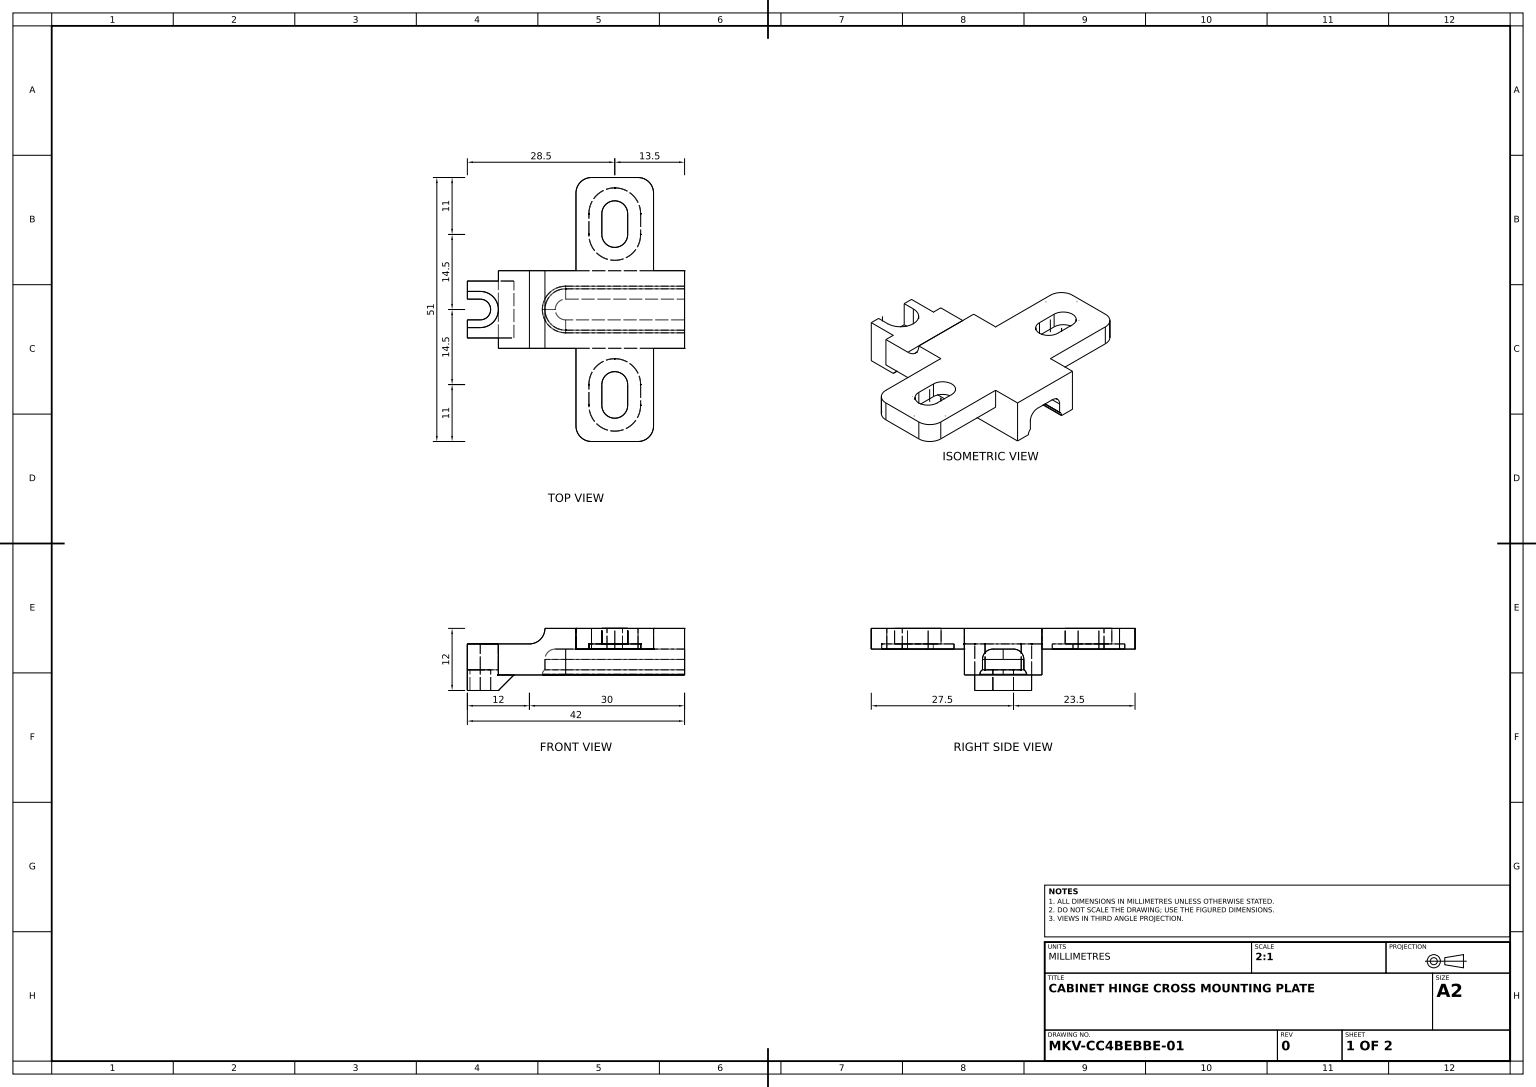
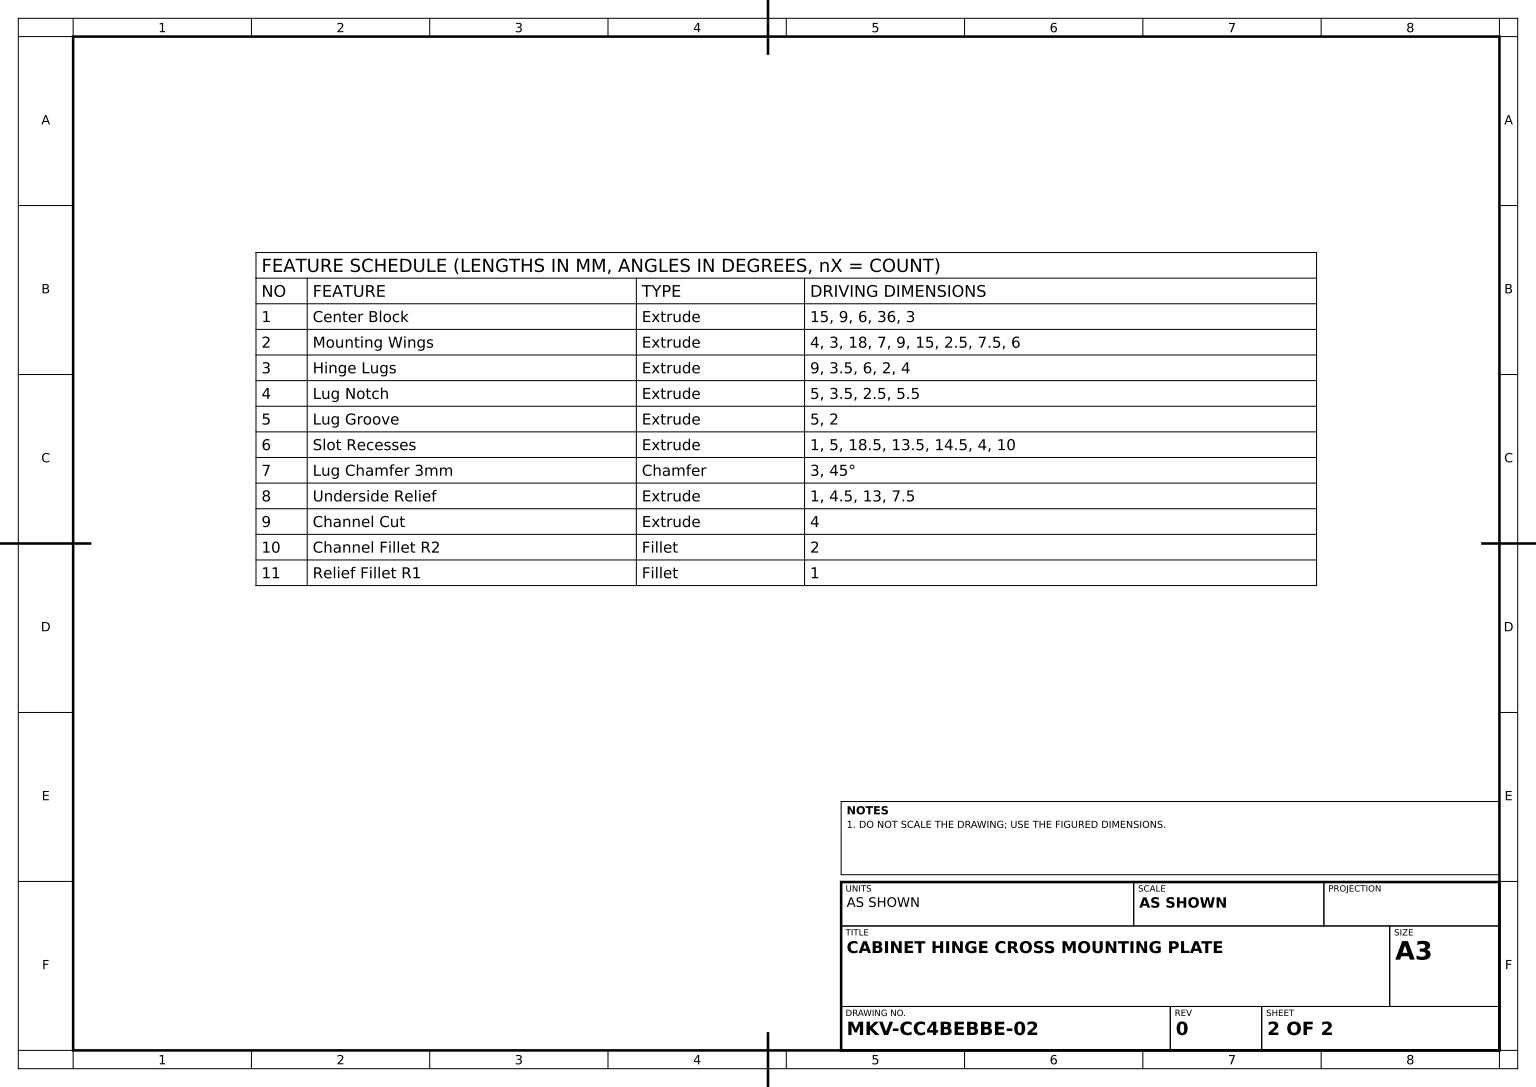
solid
v1 (-8.5,-4,18.5)
v2 (-18.5,-4,18.5)
e1 v1 v2 CIRCLE(AX(P(-13.5,-4,18.5),D(0,-1,0),D(0,0,1)),5)
v3 (-18.5,-3,18.5)
e2 v3 v2 LINE
v4 (-8.5,-3,18.5)
e3 v4 v3 CIRCLE(AX(P(-13.5,-3,18.5),D(0,-1,0),D(0,0,1)),5)
e4 v4 v1 LINE
face CYL(AX(P(-13.5,-3,18.5),D(0,-1,0),D(0,0,-1)),5) rev [e1 -e2 -e3 e4]
v5 (-9,-4,-25.5)
v6 (-18,-4,-25.5)
e5 v5 v6 LINE
v7 (-18,0,-25.5)
e6 v6 v7 LINE
v8 (-9,0,-25.5)
e7 v8 v7 LINE
e8 v5 v8 LINE
face PLANE(AX(P(-18,-4,-25.5),D(0,0,-1),D(-1,0,0))) [e5 e6 -e7 -e8]
v9 (-39.5,-8,2)
v10 (-39.5,-8,-2)
e9 v9 v10 CIRCLE(AX(P(-39.5,-8,0),D(0,1,0),D(0,0,1)),2)
v11 (-42,-8,2)
e10 v11 v9 LINE
v12 (-42,-8,3.5)
e11 v11 v12 LINE
v13 (-39.5,-8,3.5)
e12 v12 v13 LINE
v14 (-39.5,-8,-3.5)
e13 v13 v14 CIRCLE(AX(P(-39.5,-8,0),D(0,1,0),D(0,0,1)),3.5)
v15 (-42,-8,-3.5)
e14 v14 v15 LINE
v16 (-42,-8,-2)
e15 v15 v16 LINE
e16 v10 v16 LINE
face PLANE(AX(P(-39.5,-8,0),D(0,1,0),D(0,0,1))) [-e9 -e10 e11 e12 e13 e14 e15 -e16]
v17 (0,-8,-4)
v18 (0,-8.866025,-4.5)
e17 v17 v18 CIRCLE(AX(P(0,-8.866025,-3.5),D(-1,0,0),D(0,-1,0)),1)
v19 (-23,-8,-4)
e18 v19 v17 LINE
v20 (-23,-8.866025,-4.5)
e19 v20 v19 CIRCLE(AX(P(-23,-8.866025,-3.5),D(1,0,0),D(0,0,-1)),1)
e20 v18 v20 LINE
face CYL(AX(P(-23,-8.866025,-3.5),D(1,0,0),D(0,1,0)),1) rev [-e17 -e18 -e19 -e20]
v21 (-8.5,-4,14.5)
e21 v21 v1 LINE
v22 (-8.5,-3,14.5)
e22 v22 v4 LINE
e23 v22 v21 LINE
face PLANE(AX(P(-8.5,-3,14.5),D(1,0,0),D(0,0,-1))) rev [e21 -e4 -e22 e23]
v23 (-6,-4,-7.5)
v24 (-6,0,-7.5)
e24 v23 v24 LINE
v25 (0,0,-7.5)
e25 v25 v24 LINE
v26 (0,-9,-7.5)
e26 v26 v25 LINE
v27 (-36,-9,-7.5)
e27 v27 v26 LINE
v28 (-36,-3,-7.5)
e28 v28 v27 LINE
v29 (-30,-3,-7.5)
e29 v29 v28 LINE
v30 (-27,0,-7.5)
e30 v30 v29 CIRCLE(AX(P(-30,0,-7.5),D(0,0,-1),D(1,0,0)),3)
v31 (-21,0,-7.5)
e31 v31 v30 LINE
v32 (-21,-4,-7.5)
e32 v32 v31 LINE
e33 v32 v23 LINE
face PLANE(AX(P(-30,0,-7.5),D(0,0,1),D(1,0,0))) rev [e24 -e25 -e26 -e27 -e28 -e29 -e30 -e31 -e32 e33]
v33 (-11,-3,14.5)
v34 (-11,0,14.5)
e34 v33 v34 LINE
v35 (-11,-3,18.5)
e35 v33 v35 LINE
v36 (-11,0,18.5)
e36 v35 v36 LINE
e37 v36 v34 LINE
face PLANE(AX(P(-11,-4,18.5),D(1,0,0),D(0,0,-1))) rev [-e34 e35 e36 e37]
v37 (-8.5,-3,-14.5)
v38 (-18.5,-3,-14.5)
e38 v37 v38 CIRCLE(AX(P(-13.5,-3,-14.5),D(0,-1,0),D(0,0,-1)),5)
v39 (-8.5,-4,-14.5)
e39 v37 v39 LINE
v40 (-18.5,-4,-14.5)
e40 v39 v40 CIRCLE(AX(P(-13.5,-4,-14.5),D(0,-1,0),D(0,0,-1)),5)
e41 v38 v40 LINE
face CYL(AX(P(-13.5,-3,-14.5),D(0,-1,0),D(0,0,-1)),5) rev [-e38 e39 e40 -e41]
v41 (-23,-9,-4.5)
e42 v20 v41 LINE
v42 (0,-9,-4.5)
e43 v41 v42 LINE
e44 v18 v42 LINE
face PLANE(AX(P(0,-8,-4.5),D(0,0,-1),D(-1,0,0))) rev [e42 e43 -e44 e20]
v43 (-16,-3,-14.5)
v44 (-16,0,-14.5)
e45 v43 v44 LINE
v45 (-13.5,0,-12)
e46 v44 v45 CIRCLE(AX(P(-13.5,0,-14.5),D(0,1,0),D(0,0,1)),2.5)
v46 (-13.5,-3,-12)
e47 v46 v45 LINE
e48 v43 v46 CIRCLE(AX(P(-13.5,-3,-14.5),D(0,1,0),D(0,0,-1)),2.5)
face CYL(AX(P(-13.5,-4,-14.5),D(0,1,0),D(0,0,1)),2.5) rev [e45 e46 -e47 -e48]
v47 (0,-6,-4)
e49 v47 v17 LINE
e50 v42 v26 LINE
v48 (0,0,7.5)
e51 v48 v25 LINE
v49 (0,-9,7.5)
e52 v49 v48 LINE
v50 (0,-9,4.5)
e53 v49 v50 LINE
v51 (0,-8.866025,4.5)
e54 v51 v50 LINE
v52 (0,-8,4)
e55 v51 v52 CIRCLE(AX(P(0,-8.866025,3.5),D(-1,0,0),D(0,-1,0)),1)
v53 (0,-6,4)
e56 v53 v52 LINE
v54 (0,-4,2)
e57 v53 v54 CIRCLE(AX(P(0,-6,2),D(-1,0,0),D(0,-1,0)),2)
v55 (0,-4,-2)
e58 v55 v54 LINE
e59 v55 v47 CIRCLE(AX(P(0,-6,-2),D(-1,0,0),D(0,-1,0)),2)
face PLANE(AX(P(0,0,7.5),D(-1,0,0),D(0,-1,0))) rev [e49 e17 e44 e50 e26 -e51 -e52 e53 -e54 e55 -e56 e57 -e58 e59]
v56 (-18,-4,25.5)
v57 (-18,0,25.5)
e60 v56 v57 LINE
v58 (-9,-4,25.5)
e61 v56 v58 LINE
v59 (-9,0,25.5)
e62 v58 v59 LINE
e63 v57 v59 LINE
face PLANE(AX(P(-18,-4,25.5),D(0,0,1),D(1,0,0))) [-e60 e61 e62 -e63]
v60 (-6,-4,22.5)
v61 (-6,0,22.5)
e64 v60 v61 LINE
v62 (-6,-4,7.5)
e65 v60 v62 LINE
v63 (-6,0,7.5)
e66 v62 v63 LINE
e67 v61 v63 LINE
face PLANE(AX(P(-6,-4,22.5),D(1,0,0),D(0,0,-1))) [-e64 e65 e66 -e67]
v64 (-13.5,-3,9.5)
v65 (-13.5,-4,9.5)
e68 v64 v65 LINE
v66 (-18.5,-3,14.5)
e69 v66 v64 CIRCLE(AX(P(-13.5,-3,14.5),D(0,-1,0),D(0,0,1)),5)
v67 (-18.5,-4,14.5)
e70 v66 v67 LINE
e71 v67 v65 CIRCLE(AX(P(-13.5,-4,14.5),D(0,-1,0),D(0,0,1)),5)
face CYL(AX(P(-13.5,-3,14.5),D(0,-1,0),D(0,0,-1)),5) rev [-e68 -e69 e70 e71]
e72 v59 v61 CIRCLE(AX(P(-9,0,22.5),D(0,1,0),D(0,0,-1)),3)
e73 v58 v60 CIRCLE(AX(P(-9,-4,22.5),D(0,1,0),D(0,0,-1)),3)
face CYL(AX(P(-9,-4,22.5),D(0,1,0),D(0,0,1)),3) [e64 -e72 -e62 e73]
v68 (-18.5,-3,-18.5)
v69 (-13.5,-3,-23.5)
e74 v68 v69 CIRCLE(AX(P(-13.5,-3,-18.5),D(0,-1,0),D(0,0,-1)),5)
v70 (-18.5,-4,-18.5)
e75 v68 v70 LINE
v71 (-13.5,-4,-23.5)
e76 v70 v71 CIRCLE(AX(P(-13.5,-4,-18.5),D(0,-1,0),D(0,0,-1)),5)
e77 v69 v71 LINE
face CYL(AX(P(-13.5,-3,-18.5),D(0,-1,0),D(0,0,-1)),5) rev [-e74 e75 e76 -e77]
v72 (-16,0,14.5)
e78 v34 v72 CIRCLE(AX(P(-13.5,0,14.5),D(0,1,0),D(0,0,-1)),2.5)
v73 (-16,-3,14.5)
e79 v73 v72 LINE
e80 v73 v33 CIRCLE(AX(P(-13.5,-3,14.5),D(0,-1,0),D(0,0,1)),2.5)
face CYL(AX(P(-13.5,-4,14.5),D(0,1,0),D(0,0,1)),2.5) rev [e78 -e79 e80 e34]
v74 (-36,-12,-5.5)
v75 (-42,-12,-5.5)
e81 v74 v75 LINE
v76 (-42,-3,-5.5)
e82 v75 v76 LINE
v77 (-36,-3,-5.5)
e83 v77 v76 LINE
v78 (-36,-9,-5.5)
e84 v78 v77 LINE
v79 (-33,-9,-5.5)
e85 v79 v78 LINE
e86 v79 v74 LINE
face PLANE(AX(P(-36,-12,-5.5),D(0,0,-1),D(-1,0,0))) [e81 e82 -e83 -e84 -e85 e86]
v80 (-6,-4,-22.5)
e87 v23 v80 LINE
v81 (-6,0,-22.5)
e88 v80 v81 LINE
e89 v24 v81 LINE
face PLANE(AX(P(-6,-4,-22.5),D(1,0,0),D(0,0,-1))) [e87 e88 -e89 -e24]
v82 (-13.5,0,21)
e90 v82 v36 CIRCLE(AX(P(-13.5,0,18.5),D(0,1,0),D(0,0,-1)),2.5)
v83 (-13.5,-3,21)
e91 v35 v83 CIRCLE(AX(P(-13.5,-3,18.5),D(0,-1,0),D(0,0,1)),2.5)
e92 v83 v82 LINE
face CYL(AX(P(-13.5,-4,18.5),D(0,1,0),D(0,0,1)),2.5) rev [e90 -e36 e91 e92]
v84 (-11,-3,-14.5)
e93 v46 v84 CIRCLE(AX(P(-13.5,-3,-14.5),D(0,1,0),D(0,0,-1)),2.5)
v85 (-11,-3,-18.5)
e94 v84 v85 LINE
v86 (-16,-3,-18.5)
e95 v85 v86 CIRCLE(AX(P(-13.5,-3,-18.5),D(0,1,0),D(0,0,-1)),2.5)
e96 v86 v43 LINE
e97 v38 v68 LINE
v87 (-8.5,-3,-18.5)
e98 v69 v87 CIRCLE(AX(P(-13.5,-3,-18.5),D(0,-1,0),D(0,0,-1)),5)
e99 v87 v37 LINE
face PLANE(AX(P(-13.5,-3,-14.5),D(0,-1,0),D(0,0,-1))) [e48 e93 e94 e95 e96] [e97 e74 e98 e99 e38]
e100 v2 v67 LINE
e101 v65 v21 CIRCLE(AX(P(-13.5,-4,14.5),D(0,-1,0),D(0,0,1)),5)
v88 (-21,-4,22.5)
e102 v88 v56 CIRCLE(AX(P(-18,-4,22.5),D(0,1,0),D(0,0,1)),3)
v89 (-21,-4,7.5)
e103 v89 v88 LINE
e104 v62 v89 LINE
face PLANE(AX(P(-18,-4,22.5),D(0,1,0),D(0,0,1))) rev [-e100 -e1 -e21 -e101 -e71] [-e65 -e73 -e61 -e102 -e103 -e104]
v90 (-27.5,-8.866025,0)
v91 (-27,-8,0)
e105 v90 v91 CIRCLE(AX(P(-26.5,-8.866025,0),D(0,0,-1),D(-1,0,0)),1)
e106 v20 v90 CIRCLE(AX(P(-23,-8.866025,0),D(0,1,0),D(-1,0,0)),4.5)
e107 v91 v19 CIRCLE(AX(P(-23,-8,0),D(0,-1,0),D(1,0,0)),4)
face TORUS(AX(P(-23,-8.866025,0),D(0,1,0),D(-1,0,0)),3.5,1) rev [-e105 -e106 e19 -e107]
v92 (-23,-8.866025,4.5)
e108 v92 v51 LINE
v93 (-23,-8,4)
e109 v92 v93 CIRCLE(AX(P(-23,-8.866025,3.5),D(-1,0,0),D(0,0,1)),1)
e110 v52 v93 LINE
face CYL(AX(P(-23,-8.866025,3.5),D(-1,0,0),D(0,-1,0)),1) rev [-e55 -e108 e109 -e110]
v94 (-8.5,-4,-18.5)
e111 v71 v94 CIRCLE(AX(P(-13.5,-4,-18.5),D(0,-1,0),D(0,0,-1)),5)
e112 v87 v94 LINE
face CYL(AX(P(-13.5,-3,-18.5),D(0,-1,0),D(0,0,-1)),5) rev [e111 -e112 -e98 e77]
v95 (-42,-12,2)
e113 v95 v11 LINE
v96 (-39.5,-12,2)
e114 v96 v9 LINE
e115 v95 v96 LINE
face PLANE(AX(P(-42,-13,2),D(0,0,1),D(1,0,0))) rev [e113 e10 -e114 -e115]
v97 (-42,-3,3.5)
e116 v12 v97 LINE
v98 (-39.5,-3,3.5)
e117 v97 v98 LINE
e118 v13 v98 LINE
face PLANE(AX(P(-42,-8,3.5),D(0,0,1),D(1,0,0))) rev [e116 e117 -e118 -e12]
v99 (-42,-12,-2)
e119 v99 v16 LINE
v100 (-39.5,-12,-2)
e120 v100 v99 LINE
e121 v100 v10 LINE
face PLANE(AX(P(-39.5,-13,-2),D(0,0,-1),D(-1,0,0))) rev [e16 -e119 -e120 e121]
v101 (-21,0,-22.5)
e122 v7 v101 CIRCLE(AX(P(-18,0,-22.5),D(0,1,0),D(0,0,-1)),3)
v102 (-21,-4,-22.5)
e123 v6 v102 CIRCLE(AX(P(-18,-4,-22.5),D(0,1,0),D(0,0,-1)),3)
e124 v102 v101 LINE
face CYL(AX(P(-18,-4,-22.5),D(0,1,0),D(0,0,1)),3) [-e122 -e6 e123 e124]
e125 v81 v8 CIRCLE(AX(P(-9,0,-22.5),D(0,1,0),D(0,0,-1)),3)
e126 v80 v5 CIRCLE(AX(P(-9,-4,-22.5),D(0,1,0),D(0,0,-1)),3)
face CYL(AX(P(-9,-4,-22.5),D(0,1,0),D(0,0,1)),3) [-e125 -e88 e126 e8]
v103 (-21,0,22.5)
e127 v88 v103 LINE
e128 v103 v57 CIRCLE(AX(P(-18,0,22.5),D(0,1,0),D(0,0,1)),3)
face CYL(AX(P(-18,-4,22.5),D(0,1,0),D(0,0,1)),3) [-e127 e102 e60 -e128]
e129 v90 v92 CIRCLE(AX(P(-23,-8.866025,0),D(0,1,0),D(-1,0,0)),4.5)
e130 v93 v91 CIRCLE(AX(P(-23,-8,0),D(0,-1,0),D(1,0,0)),4)
face TORUS(AX(P(-23,-8.866025,0),D(0,1,0),D(-1,0,0)),3.5,1) rev [-e109 -e129 e105 -e130]
v104 (-23,-9,4.5)
e131 v104 v41 CIRCLE(AX(P(-23,-9,0),D(0,-1,0),D(1,0,0)),4.5)
e132 v50 v104 LINE
v105 (-36,-9,7.5)
e133 v105 v49 LINE
v106 (-36,-9,5.5)
e134 v105 v106 LINE
v107 (-33,-9,5.5)
e135 v106 v107 LINE
e136 v107 v79 LINE
e137 v78 v27 LINE
face PLANE(AX(P(0,-9,7.5),D(0,1,0),D(-1,0,0))) rev [-e131 -e132 -e53 -e133 e134 e135 e136 e85 e137 e27 -e50 -e43]
v108 (-23,-4,2)
v109 (-25,-4,0)
e138 v108 v109 CIRCLE(AX(P(-23,-4,0),D(0,-1,0),D(1,0,0)),2)
v110 (-23,-6,4)
e139 v110 v108 CIRCLE(AX(P(-23,-6,2),D(-1,0,0),D(0,0,1)),2)
v111 (-27,-6,0)
e140 v111 v110 CIRCLE(AX(P(-23,-6,0),D(0,1,0),D(1,0,0)),4)
e141 v109 v111 CIRCLE(AX(P(-25,-6,0),D(0,0,1),D(1,0,0)),2)
face TORUS(AX(P(-23,-6,0),D(0,-1,0),D(1,0,0)),2,2) rev [-e138 -e139 -e140 -e141]
e142 v110 v53 LINE
e143 v54 v108 LINE
face CYL(AX(P(-23,-6,2),D(-1,0,0),D(0,-1,0)),2) rev [-e57 -e142 e139 -e143]
v112 (-23,-6,-4)
e144 v112 v111 CIRCLE(AX(P(-23,-6,0),D(0,1,0),D(1,0,0)),4)
v113 (-23,-4,-2)
e145 v112 v113 CIRCLE(AX(P(-23,-6,-2),D(1,0,0),D(0,0,-1)),2)
e146 v109 v113 CIRCLE(AX(P(-23,-4,0),D(0,-1,0),D(1,0,0)),2)
face TORUS(AX(P(-23,-6,0),D(0,-1,0),D(1,0,0)),2,2) rev [e141 -e144 e145 -e146]
v114 (-11,0,-14.5)
e147 v84 v114 LINE
e148 v45 v114 CIRCLE(AX(P(-13.5,0,-14.5),D(0,1,0),D(0,0,1)),2.5)
face CYL(AX(P(-13.5,-4,-14.5),D(0,1,0),D(0,0,1)),2.5) rev [-e147 -e93 e47 e148]
v115 (-36,-3,5.5)
e149 v106 v115 LINE
v116 (-42,-3,5.5)
e150 v116 v115 LINE
v117 (-42,-12,5.5)
e151 v117 v116 LINE
v118 (-36,-12,5.5)
e152 v117 v118 LINE
e153 v118 v107 LINE
face PLANE(AX(P(-39.5,-12,5.5),D(0,0,1),D(1,0,0))) [-e135 e149 -e150 -e151 e152 e153]
v119 (-39.5,-3,-3.5)
e154 v14 v119 LINE
v120 (-42,-3,-3.5)
e155 v119 v120 LINE
e156 v15 v120 LINE
face PLANE(AX(P(-39.5,-8,-3.5),D(0,0,-1),D(-1,0,0))) rev [-e14 e154 e155 -e156]
v121 (-36,-3,7.5)
e157 v121 v115 LINE
e158 v121 v105 LINE
face PLANE(AX(P(-36,-9,7.5),D(1,0,0),D(0,0,-1))) rev [e157 -e149 -e134 -e158]
e159 v110 v93 LINE
face PLANE(AX(P(-23,-4,4),D(0,0,1),D(1,0,0))) rev [e110 -e159 e142 e56]
e160 v92 v104 LINE
face CYL(AX(P(-23,-8,0),D(0,-1,0),D(1,0,0)),4.5) rev [e129 e160 e131 -e42 e106]
v122 (-16,-3,18.5)
e161 v83 v122 CIRCLE(AX(P(-13.5,-3,18.5),D(0,-1,0),D(0,0,1)),2.5)
v123 (-16,0,18.5)
e162 v122 v123 LINE
e163 v123 v82 CIRCLE(AX(P(-13.5,0,18.5),D(0,1,0),D(0,0,-1)),2.5)
face CYL(AX(P(-13.5,-4,18.5),D(0,1,0),D(0,0,1)),2.5) rev [-e92 e161 e162 e163]
e164 v102 v32 LINE
e165 v40 v70 LINE
e166 v94 v39 LINE
face PLANE(AX(P(-18,-4,-22.5),D(0,-1,0),D(0,0,-1))) [-e33 -e164 -e123 -e5 -e126 -e87] [-e165 -e40 -e166 -e111 -e76]
e167 v64 v22 CIRCLE(AX(P(-13.5,-3,14.5),D(0,-1,0),D(0,0,1)),5)
face CYL(AX(P(-13.5,-3,14.5),D(0,-1,0),D(0,0,-1)),5) rev [e68 e101 -e23 -e167]
e168 v3 v66 LINE
face PLANE(AX(P(-18.5,-3,14.5),D(-1,0,0),D(0,0,1))) rev [e2 e100 -e70 -e168]
v124 (-30,-3,7.5)
e169 v124 v121 LINE
e170 v124 v29 LINE
e171 v77 v28 LINE
e172 v76 v120 LINE
e173 v98 v119 CIRCLE(AX(P(-39.5,-3,0),D(0,1,0),D(0,0,1)),3.5)
e174 v97 v116 LINE
face PLANE(AX(P(-36,-3,7.5),D(0,-1,0),D(0,0,-1))) rev [-e157 -e169 e170 e29 -e171 e83 e172 -e155 -e173 -e117 e174 e150]
e175 v96 v100 CIRCLE(AX(P(-39.5,-12,0),D(0,1,0),D(0,0,1)),2)
face CYL(AX(P(-39.5,-13,0),D(0,1,0),D(0,0,1)),2) rev [e9 -e121 -e175 e114]
face CYL(AX(P(-39.5,-8,0),D(0,1,0),D(0,0,1)),3.5) rev [e173 -e154 -e13 e118]
e176 v112 v19 LINE
e177 v47 v112 LINE
face PLANE(AX(P(0,-4,-4),D(0,0,-1),D(-1,0,0))) rev [e176 e18 -e49 e177]
v125 (-16,0,-18.5)
e178 v86 v125 LINE
e179 v125 v44 LINE
face PLANE(AX(P(-16,-4,-18.5),D(-1,0,0),D(0,0,1))) rev [e178 e179 -e45 -e96]
v126 (-11,0,-18.5)
e180 v114 v126 LINE
e181 v85 v126 LINE
face PLANE(AX(P(-11,-4,-18.5),D(1,0,0),D(0,0,-1))) rev [-e94 e147 e180 -e181]
v127 (-27,0,7.5)
e182 v127 v124 CIRCLE(AX(P(-30,0,7.5),D(0,0,-1),D(1,0,0)),3)
e183 v127 v30 LINE
face CYL(AX(P(-30,0,7.5),D(0,0,-1),D(-1,0,0)),3) rev [-e182 e183 e30 -e170]
e184 v122 v73 LINE
e185 v72 v123 LINE
face PLANE(AX(P(-16,-4,18.5),D(-1,0,0),D(0,0,1))) rev [e184 e79 e185 -e162]
face PLANE(AX(P(-36,-9,7.5),D(1,0,0),D(0,0,-1))) rev [e28 -e137 e84 e171]
face PLANE(AX(P(-23,-8,4.5),D(0,0,1),D(1,0,0))) rev [-e160 e108 e54 e132]
face CYL(AX(P(-23,-4,0),D(0,-1,0),D(1,0,0)),4) rev [-e176 e144 e140 e159 e130 e107]
e186 v48 v63 LINE
v128 (-21,0,7.5)
e187 v89 v128 LINE
e188 v128 v127 LINE
face PLANE(AX(P(-30,0,7.5),D(0,0,1),D(1,0,0))) [e182 e169 e158 e133 e52 e186 -e66 e104 e187 e188]
e189 v128 v103 LINE
face PLANE(AX(P(-21,-4,7.5),D(-1,0,0),D(0,0,1))) [e127 -e189 -e187 e103]
e190 v101 v31 LINE
face PLANE(AX(P(-21,-4,-7.5),D(-1,0,0),D(0,0,1))) [-e190 -e124 e164 e32]
e191 v118 v74 LINE
face PLANE(AX(P(-33,-9,7.5),D(-0.707106781,0.707106781,0),D(0,0,-1))) rev [e191 -e86 -e136 -e153]
e192 v126 v125 CIRCLE(AX(P(-13.5,0,-18.5),D(0,1,0),D(0,0,1)),2.5)
face PLANE(AX(P(-27,0,7.5),D(0,-1,0),D(0,0,-1))) rev [-e37 -e90 -e163 -e185 -e78] [-e148 -e46 -e179 -e192 -e180] [e128 e63 e72 e67 -e186 e51 e25 e89 e125 e7 e122 e190 e31 -e183 -e188 e189]
e193 v113 v55 LINE
face CYL(AX(P(-23,-6,-2),D(1,0,0),D(0,1,0)),2) rev [-e59 -e193 -e145 -e177]
face PLANE(AX(P(-18.5,-3,-14.5),D(-1,0,0),D(0,0,1))) rev [e165 -e75 -e97 e41]
face PLANE(AX(P(-23,-4,0),D(0,-1,0),D(1,0,0))) [e146 e193 e58 e143 e138]
e194 v75 v99 LINE
face PLANE(AX(P(-42,-12,5.5),D(-1,0,0),D(0,0,1))) [-e15 e156 -e172 -e82 e194 e119]
e195 v95 v117 LINE
face PLANE(AX(P(0,-12,0),D(0,1,0),D(0,0,1))) rev [-e194 -e81 -e191 -e152 -e195 e115 e175 e120]
face PLANE(AX(P(-8.5,-3,-14.5),D(1,0,0),D(0,0,-1))) rev [e166 -e39 -e99 e112]
face PLANE(AX(P(-13.5,-3,18.5),D(0,1,0),D(0,0,1))) rev [e167 e22 e3 e168 e69] [-e161 -e91 -e35 -e80 -e184]
face CYL(AX(P(-13.5,-4,-18.5),D(0,1,0),D(0,0,1)),2.5) rev [e181 e192 -e178 -e95]
face PLANE(AX(P(-42,-12,5.5),D(-1,0,0),D(0,0,1))) [e151 -e174 -e116 -e11 -e113 e195]
